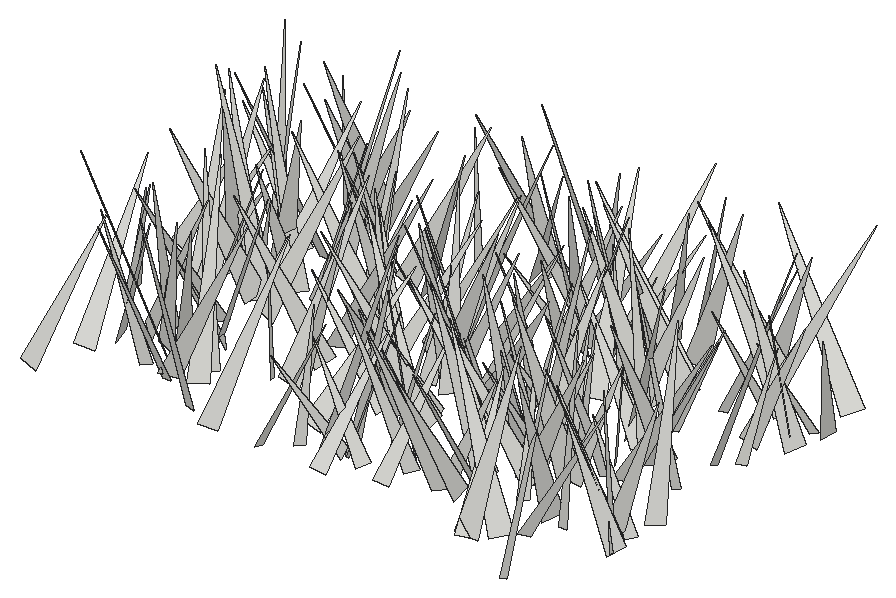
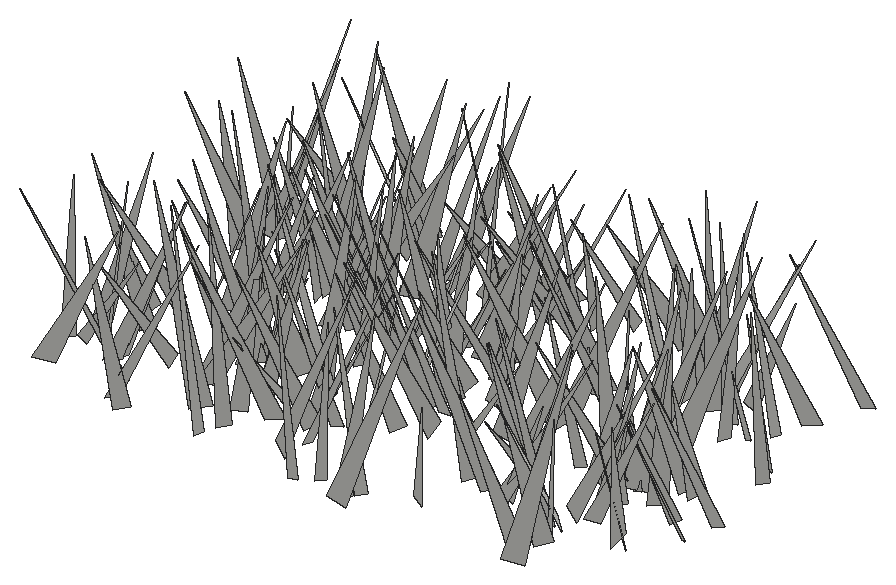
# SketchUp Ruby script. Lengths in inches.
U = 1.inch
M = Sketchup.active_model
def pt(a) = Geom::Point3d.new(a.map { |v| v * U })
def face(e, loops, mat)
  f = e.add_face(loops[0].map { |a| pt(a) })
  loops[1..].each { |l| e.add_face(l.map { |a| pt(a) }).erase! }
  f.material = f.back_material = mat if mat
  f
end
# faces: each face lists its corners as indices into pts; further lists are holes
def faces(e, pts, list, mat = nil) = list.each { |f| face(e, (f[0].is_a?(Array) ? f : [f]).map { |l| l.map { |i| pts[i] } }, mat) }
# xy, xz, yz: faces in a plane at the given z, y or x. An outline is a flat list of corners, or four numbers for a rectangle; further outlines are holes
def ring(l) = l.size == 4 ? [[l[0], l[1]], [l[2], l[1]], [l[2], l[3]], [l[0], l[3]]] : l.each_slice(2).to_a
def flat(e, list, mat, &to3) = list.each { |f| face(e, (f[0].is_a?(Array) ? f : [f]).map { |l| ring(l).map { |u, v| to3.(u, v) } }, mat) }
def xy(e, z, list, mat = nil) = flat(e, list, mat) { |x, y| [x, y, z] }
def xz(e, y, list, mat = nil) = flat(e, list, mat) { |x, z| [x, y, z] }
def yz(e, x, list, mat = nil) = flat(e, list, mat) { |y, z| [x, y, z] }
def lines(e, pts, list) = list.each { |a, b| e.add_line(pt(pts[a]), pt(pts[b])) }
# prism: a flat outline (further loops are holes) pulled along v
def prism(e, loops, v, mat = nil)
  f = face(e, loops, mat); d = Geom::Vector3d.new(v.map { |x| x * U })
  f.pushpull(f.normal.samedirection?(d) ? d.length : -d.length)
end
def box(e, o, s, mat = nil) = prism(e, [[o, [o[0] + s[0], o[1], o[2]], [o[0] + s[0], o[1] + s[1], o[2]], [o[0], o[1] + s[1], o[2]]]], [0, 0, s[2]], mat)
def at(x, y, z, deg = 0) = Geom::Transformation.translation(pt([x, y, z])) * Geom::Transformation.rotation(ORIGIN, Z_AXIS, deg.degrees)
def axes(o, x, y, z) = Geom::Transformation.new([*x, 0, *y, 0, *z, 0, *pt(o).to_a, 1])
def part(name) = M.definitions.add(name)
# library, detail: a bought-in or finely detailed component or shape, given as its bounding box
def library(name, o, s) = part(name).tap { |d| box(d.entities, o, s) }
def detail(e, o, s) = box(e.add_group.entities, o, s)
def put(e, d, t, mat = nil) = e.add_instance(d, t).tap { |i| i.material = mat if mat }
def group(e, t, mat = nil) = e.add_group.tap { |g| g.transformation = t; g.material = mat if mat }.entities
root = M.entities
c1 = part("fur_instance\#9")
p = [[0.8125,0,1.79],[0.67,-0.02,1.48],[0,-0.11,0],[0,0.11,0]]
faces(c1.entities,p,[[0,1,2,3]])
put(root,c1,axes([534.58,361.02,-21.66],[-6.04066,-0.63869,2.51357],[0.73038,5.69455,3.20222],[2.48847,-3.22176,5.16172]))
put(root,c1,axes([538.41,356.86,-21.66],[-1.59502,6.99566,2.35908],[7.02793,2.17795,-1.70682],[2.26111,-1.83463,6.96922]))
put(root,c1,axes([525,360.51,-21.66],[-5.02387,-1.18033,0.42976],[-0.88594,4.58548,2.23734],[0.8905,-2.09699,4.65046]))
put(root,c1,axes([538.34,359.93,-21.66],[-2.23247,-5.83337,0.18602],[-5.6892,2.13065,-1.46288],[-1.30221,0.692,6.07224]))
put(root,c1,axes([543.93,353.875,-21.66],[4.35175,7.0169,0.44581],[6.16578,-4.0605,3.72408],[-3.37917,1.6275,7.36925]))
put(root,c1,axes([500.89,356.83,-21.66],[0.65701,6.39206,0.99008],[6.12037,-0.29236,-2.17392],[2.09278,-1.15171,6.04683]))
put(root,c1,axes([533.23,360.72,-21.66],[1.95168,-6.84621,1.26966],[-6.52036,-2.2596,-2.16121],[-2.44285,0.56154,6.78298]))
put(root,c1,axes([513.05,358.93,-21.66],[-3.81075,-5.76969,1.72606],[-6.01138,3.52106,-1.50194],[-0.36316,2.25903,6.74947]))
put(root,c1,axes([540.23,358.26,-21.66],[-4.97351,5.86998,1.15657],[5.9442,4.67754,1.82131],[-0.6788,-2.04794,7.47498]))
put(root,c1,axes([538.38,356.68,-21.66],[-4.13598,4.27474,0.09369],[4.07434,3.97972,-1.71759],[1.29691,1.13001,5.6947]))
put(root,c1,axes([519.9,357.75,-21.66],[4.92859,0.75105,0.39032],[0.57555,-4.66461,1.7081],[-0.62062,1.63853,4.68375]))
put(root,c1,axes([541.375,362.4,-21.66],[6.17469,-3.94346,0.96595],[-3.5616,-6.10514,-2.15707],[-1.94909,-1.33681,7.00177]))
put(root,c1,axes([527.08,360,-21.66],[-3.88127,2.88585,0.74535],[2.95869,3.58243,1.53633],[-0.36036,-1.66913,4.58608]))
put(root,c1,axes([509.43,361.02,-21.66],[-2.97,-5.19915,0.68344],[-5.09037,2.66981,-1.8109],[-1.25951,1.46972,5.70725]))
put(root,c1,axes([547.59,361.41,-21.66],[-5.95975,2.47486,1.75961],[2.91321,5.75356,1.77469],[0.85695,-2.34763,6.20435]))
put(root,c1,axes([546.71,363.14,-21.66],[-5.73536,-5.62008,0.65862],[-5.46135,5.74328,1.44982],[1.48081,-0.58562,7.89796]))
put(root,c1,axes([525.1,357.56,-21.66],[-2.44099,4.81015,0.04297],[4.37742,2.2412,-2.21652],[1.99437,0.96814,4.91762]))
put(root,c1,axes([521.98,359.56,-21.66],[-4.57761,1.25738,1.06742],[0.91701,4.55759,-1.43608],[1.37093,1.14988,4.52473]))
put(root,c1,axes([528.41,363.76,-21.66],[-4.91582,-6.36103,2.07601],[-5.8042,5.33544,2.60426],[3.32923,-0.09063,7.60565]))
put(root,c1,axes([515.68,357.57,-21.66],[-5.17652,4.83446,1.05401],[3.91261,4.93311,-3.41105],[3.02894,1.88989,6.20751]))
put(root,c1,axes([527.79,361.93,-21.66],[5.79589,4.16761,1.50359],[4.42839,-5.37215,-2.17978],[0.13803,-2.64446,6.79779]))
put(root,c1,axes([508.77,363.5,-21.66],[7.2919,-1.58164,0.56037],[-1.39543,-7.10365,-1.89164],[-0.93186,-1.73896,7.21769]))
put(root,c1,axes([541.37,359.32,-21.66],[5.52796,-0.81869,0.7417],[-1.07099,-4.89962,2.57397],[-0.27083,2.66498,4.96017]))
put(root,c1,axes([530.12,361.35,-21.66],[-1.81659,5.58818,1.87966],[5.39696,0.78429,2.88421],[-2.37355,-2.49359,5.11948]))
put(root,c1,axes([509.28,361.95,-21.66],[-6.03257,-5.76703,0.56772],[-5.59645,5.58532,-2.7307],[-1.50355,2.34912,7.8863]))
put(root,c1,axes([509.28,361.45,-21.66],[5.54301,-4.89223,1.08245],[-4.92161,-5.01325,2.54471],[0.93987,2.60075,6.94141]))
put(root,c1,axes([529.46,358.88,-21.66],[-3.68567,4.23937,0.30212],[3.60627,3.33103,-2.74713],[2.24908,1.60613,4.89997]))
put(root,c1,axes([507.11,361.72,-21.66],[-0.49335,5.1966,1.87912],[5.02115,-0.36617,2.33091],[-2.30734,-1.90798,4.67065]))
put(root,c1,axes([524.16,359.375,-21.66],[7.79418,1.63756,2.08164],[0.8535,-7.67768,2.8441],[-2.50726,2.47704,7.43922]))
put(root,c1,axes([547.46,361.1875,-21.66],[-5.30333,-1.20318,1.41609],[-1.56427,5.2022,-1.4382],[1.00301,1.75149,5.24448]))
put(root,c1,axes([503.37,363.69,-21.66],[6.27835,0.76334,0.54412],[0.88551,-6.03847,-1.74618],[-0.30762,-1.80294,6.07875]))
put(root,c1,axes([506.75,364.37,-21.66],[-0.2881,-6.79413,1.19024],[-6.52945,0.65262,2.14482],[2.22333,1.03623,6.45314]))
put(root,c1,axes([532.37,362.93,-21.66],[1.52627,-4.48364,1.33128],[-4.39877,-0.90019,2.01128],[1.58937,1.81423,4.28804]))
put(root,c1,axes([545.87,363.15,-21.66],[3.29636,-5.4576,1.30622],[-5.51274,-2.86598,1.93739],[1.04942,2.08768,6.07437]))
put(root,c1,axes([525.49,360.79,-21.66],[-6.79191,0.51616,3.38033],[-0.49773,7.28774,-2.11287],[3.3831,2.10844,6.47551]))
put(root,c1,axes([534.21,364.12,-21.66],[4.0303,-5.81988,3.12764],[-5.66664,-4.92868,-1.86917],[-3.39741,1.31665,6.82792]))
put(root,c1,axes([525.58,360.23,-21.66],[4.27823,3.00126,0.70858],[2.21616,-3.83495,2.86263],[-2.14435,2.02448,4.3722]))
put(root,c1,axes([547.22,363.49,-21.66],[-1.85647,3.95367,0.8299],[3.82368,1.42492,1.76516],[-1.30372,-1.4508,3.99527]))
put(root,c1,axes([542.79,361.7,-21.66],[2.80201,6.02167,1.40008],[5.6342,-3.12002,2.14317],[-2.54489,-0.27744,6.28638]))
put(root,c1,axes([502.4,360.99,-21.66],[-2.48989,6.58556,0.19317],[6.42005,2.47161,-1.51018],[1.47984,0.3578,6.87667]))
put(root,c1,axes([536.97,365.12,-21.66],[3.33833,-6.51025,0.54896],[-6.14625,-2.92038,2.74304],[2.21549,1.70799,6.78259]))
put(root,c1,axes([537.54,365.03,-21.66],[-4.43221,4.72995,1.58971],[4.78005,3.41433,3.16821],[-1.43205,-3.24253,5.65503]))
put(root,c1,axes([504.45,365.29,-21.66],[5.46808,5.3055,1.78388],[5.41419,-4.38056,-3.56761],[1.42026,-3.72732,6.73205]))
put(root,c1,axes([505.75,366.23,-21.66],[6.82649,-0.20783,2.36031],[0.47416,-6.93274,-1.9818],[-2.32152,-2.02711,6.5358]))
put(root,c1,axes([524.76,367.15,-21.66],[3.41213,-4.67618,0.33772],[-4.46229,-3.36731,-1.54031],[-1.43828,-0.64649,5.58003]))
put(root,c1,axes([539.12,367.1,-21.66],[5.28612,-6.00356,2.19792],[-5.60526,-5.72373,-2.15328],[-3.07484,0.113,7.70384]))
put(root,c1,axes([536.71,367.59,-21.66],[-4.92711,-3.11526,0.5387],[-2.69685,4.66208,2.29422],[1.64986,-1.68274,5.3589]))
put(root,c1,axes([509.4375,367.28,-21.66],[-3.6044,-3.37024,0.34721],[-3.01204,3.4196,1.92476],[1.55135,-1.19103,4.54373]))
put(root,c1,axes([538.32,363.05,-21.66],[-4.43133,1.84787,0.51045],[1.62369,4.30117,-1.47494],[1.01922,1.18203,4.56901]))
put(root,c1,axes([521.04,362.04,-21.66],[-1.51427,6.54379,0.36236],[5.84338,1.51647,-2.96661],[2.96773,0.35306,6.02606]))
put(root,c1,axes([511.43,361.89,-21.66],[-6.67493,4.02137,0.12146],[3.83511,6.43107,-2.16198],[1.21576,1.79188,7.48679]))
put(root,c1,axes([527.21,367.38,-21.66],[-8.16776,0.06376,0.0825],[0.08376,7.86119,2.21763],[0.06209,-2.2183,7.8612]))
put(root,c1,axes([539.56,364.4,-21.66],[-6.70794,-1.60484,0.19836],[-1.59675,6.44001,-1.8942],[-0.25542,1.88735,6.63204]))
put(root,c1,axes([508.95,367.23,-21.66],[8.07507,1.50255,0.4439],[1.56674,-7.73574,-2.31627],[0.00564,-2.35841,7.88031]))
put(root,c1,axes([522.47,369.46,-21.66],[4.86562,-4.5964,0.06859],[-4.19123,-4.47675,-2.68294],[-1.88818,-1.90726,6.13213]))
put(root,c1,axes([507.2,369.33,-21.66],[2.70234,-6.75975,0.1599],[-6.39067,-2.60962,-2.31767],[-2.20886,-0.71979,6.90111]))
put(root,c1,axes([511.02,363.67,-21.66],[-7.30125,2.0292,0.54339],[1.84392,7.1322,-1.85816],[1.00641,1.65384,7.34664]))
put(root,c1,axes([533.92,368.34,-21.66],[4.85347,-3.26157,0.26621],[-3.0891,-4.72355,-1.55255],[-1.07988,-1.1468,5.6377]))
put(root,c1,axes([516.47,366.8,-21.66],[3.82304,5.79974,2.60132],[6.29108,-3.01834,-2.51622],[0.9089,-3.50316,6.47466]))
put(root,c1,axes([523.32,366.76,-21.66],[-5.14523,1.96025,0.06602],[1.88898,4.90265,1.64806],[-0.52792,-1.56261,5.25356]))
put(root,c1,axes([514.91,365.48,-21.66],[-3.90269,-1.36809,1.23152],[-1.73858,3.68797,-1.41263],[0.60468,1.77384,3.88679]))
put(root,c1,axes([536.375,366.77,-21.66],[2.73482,-5.11249,1.4467],[-5.08402,-2.04521,2.38319],[1.54377,2.32148,5.28557]))
put(root,c1,axes([516.375,369.32,-21.66],[-6.66712,2.68909,2.42043],[3.53397,5.92752,3.14894],[0.77508,-3.89533,6.46266]))
put(root,c1,axes([500.76,367.66,-21.66],[-1.89095,-4.65132,2.366],[-4.60338,2.67208,1.57395],[2.45798,1.42605,4.76793]))
put(root,c1,axes([539.4,366.96,-21.66],[-0.77235,4.89048,2.70767],[4.92537,1.88806,-2.00519],[2.64368,-2.08884,4.52687]))
put(root,c1,axes([526.59,368.86,-21.66],[-3.56897,-0.50146,0.42511],[-0.28446,3.29362,1.49696],[0.59267,-1.43888,3.27843]))
put(root,c1,axes([533.05,368.97,-21.66],[-6.0404,2.2493,3.21945],[3.13358,6.3206,1.46334],[2.36747,-2.62704,6.2773]))
put(root,c1,axes([499.96,369.28,-21.66],[5.73315,-1.08828,0.33068],[-0.98004,-5.58896,-1.40205],[-0.57725,-1.3198,5.66459]))
put(root,c1,axes([516.2,365.64,-21.66],[0.38295,8.08113,1.09098],[7.9956,-0.1576,-1.6392],[1.60161,-1.14545,7.92239]))
put(root,c1,axes([547.3125,365.94,-21.66],[-5.92088,3.75972,1.43779],[3.50525,6.07307,-1.44586],[1.97886,0.49178,6.86307]))
put(root,c1,axes([540.71,368.97,-21.66],[-1.01411,-6.0227,1.51425],[-5.97973,0.53295,-1.88497],[-1.67593,1.7428,5.80932]))
put(root,c1,axes([536.11,370.92,-21.66],[3.38656,-3.48151,1.0277],[-2.77448,-3.38882,-2.33752],[-2.3408,-1.02022,4.25743]))
put(root,c1,axes([525.11,367.82,-21.66],[-3.78872,6.01371,0.63065],[5.87535,3.48538,2.06137],[-1.42923,-1.61377,6.8022]))
put(root,c1,axes([530.73,369.39,-21.66],[-3.83855,4.56526,0.77541],[4.17711,2.97899,3.13921],[-1.99865,-2.54191,5.07163]))
put(root,c1,axes([538.84,367.01,-21.66],[-5.03448,1.97141,0.87824],[1.57247,4.87743,-1.93439],[1.47821,1.52579,5.04882]))
put(root,c1,axes([541.9,369.2,-21.66],[6.07863,-4.42165,0.21276],[-4.21796,-5.67554,2.55792],[1.3435,2.18706,7.06807]))
put(root,c1,axes([539.06,367.86,-21.66],[-5.01986,0.40192,1.5189],[-0.17545,4.90978,-1.87904],[1.56135,1.84392,4.67223]))
put(root,c1,axes([526.98,372.4,-21.66],[-6.21102,-4.85766,0.88936],[-4.64444,6.23147,1.60082],[1.67841,-0.73247,7.72082]))
put(root,c1,axes([539.78,371.12,-21.66],[4.17117,1.8451,1.43695],[2.27213,-3.89306,-1.59669],[-0.55375,-2.07548,4.27243]))
put(root,c1,axes([530.96,368.66,-21.66],[-6.11447,-3.98639,0.59028],[-3.68819,5.10346,-3.73879],[-1.62389,3.41906,6.26894]))
put(root,c1,axes([505.19,371.05,-21.66],[6.89965,2.05968,0.48381],[2.11498,-6.67017,-1.76557],[0.05673,-1.82978,6.98071]))
put(root,c1,axes([528.01,372.39,-21.66],[1.13503,-7.67663,0.6742],[-6.50823,-0.58999,4.2389],[4.12651,1.18099,6.50005]))
put(root,c1,axes([515.25,367.24,-21.66],[6.25178,5.32919,0.93445],[4.93149,-6.20008,2.36594],[-2.22574,1.23164,7.86685]))
put(root,c1,axes([542.48,373.15,-21.66],[3.73251,-5.71066,0.85994],[-5.41751,-3.81707,-1.83396],[-2.00044,-0.31799,6.57114]))
put(root,c1,axes([534.16,367.86,-21.66],[3.4696,4.95294,0.18512],[4.68916,-3.35343,1.83583],[-1.60551,0.90933,5.7619]))
put(root,c1,axes([507.08,373.47,-21.66],[-7.12654,1.94071,2.81889],[3.04033,6.57978,3.15641],[1.57127,-3.9294,6.67765]))
put(root,c1,axes([522.04,369.34,-21.66],[-6.81045,0.95525,0.6863],[0.79996,6.71798,-1.4123],[0.86231,1.31226,6.73054]))
put(root,c1,axes([523.93,373.36,-21.66],[5.76412,-4.56343,1.38579],[-4.26746,-5.90574,-1.69745],[-2.12934,-0.51736,7.15322]))
put(root,c1,axes([535.9,367.22,-21.66],[7.29611,1.84526,3.54482],[-0.04664,-7.33917,3.91643],[-3.99607,3.45479,6.4265]))
put(root,c1,axes([534.38,369.73,-21.66],[-2.83058,6.09964,1.95872],[5.76034,3.3604,-2.14023],[2.80369,-0.74599,6.37473]))
put(root,c1,axes([531.0625,373.53,-21.66],[5.81845,-0.62274,2.18855],[-0.03101,-6.03017,-1.6334],[-2.27522,-1.51035,5.61909]))
put(root,c1,axes([523.18,373.42,-21.66],[5.01421,-5.55154,0.43768],[-5.45899,-4.78379,1.86233],[1.10028,1.565,7.24525]))
put(root,c1,axes([545.39,370.61,-21.66],[-6.80362,-1.51626,0.05987],[-1.39466,6.13985,-2.9915],[-0.59797,2.93174,6.29597]))
put(root,c1,axes([520.3,370.92,-21.66],[1.42855,6.69806,0.59183],[6.31436,-1.12829,-2.47201],[2.31152,-1.05735,6.38701]))
put(root,c1,axes([515.41,371.52,-21.66],[7.23014,-2.66142,0.8801],[-2.79977,-6.73645,2.62947],[0.1379,2.76941,7.24182]))
put(root,c1,axes([538.4,374.62,-21.66],[7.85727,-0.11013,0.63762],[0.0287,-7.70188,-1.68396],[-0.64642,-1.6806,7.67549]))
put(root,c1,axes([527.13,372.38,-21.66],[4.92095,5.18553,0.33695],[5.09859,-4.72846,-1.69263],[1.00379,-1.4039,6.94554]))
put(root,c1,axes([525.42,371.26,-21.66],[-6.65914,2.85732,1.17721],[2.6023,6.69305,-1.52492],[1.66678,0.96593,7.084]))
put(root,c1,axes([541.93,371.97,-21.66],[5.39304,-0.33096,0.39775],[-0.43435,-5.15892,1.59671],[-0.28121,1.6213,5.16187]))
put(root,c1,axes([509.06,371.89,-21.66],[1.74287,7.71217,1.36191],[7.45298,-1.20484,-2.71503],[2.4053,-1.85492,7.42588]))
put(root,c1,axes([503.64,375.98,-21.66],[7.57168,-2.77915,1.4038],[-2.39268,-7.55557,-2.05259],[-1.99233,-1.48808,7.80006]))
put(root,c1,axes([539.83,373.61,-21.66],[-4.53112,4.00144,0.54603],[3.94801,4.21612,1.86503],[-0.85024,-1.74745,5.75015]))
put(root,c1,axes([526.09,373.76,-21.66],[-5.87124,-3.56524,0.53214],[-3.58838,5.68376,-1.51131],[-0.34307,1.5651,6.70063]))
put(root,c1,axes([520.78,372.16,-21.66],[-1.18961,5.30841,0.21099],[4.92708,1.02155,2.07828],[-1.98686,-0.64508,5.02744]))
put(root,c1,axes([510.92,375.14,-21.66],[-0.06945,-5.66946,1.63507],[-5.27402,0.7929,2.5253],[2.64594,1.43164,5.07647]))
put(root,c1,axes([531.5,377.09,-21.66],[5.49992,-4.64771,0.52674],[-4.40214,-5.41809,-1.84207],[-1.58109,-1.08206,6.96111]))
put(root,c1,axes([505.89,375.27,-21.66],[-0.58442,-4.16845,1.10453],[-3.96593,0.95723,1.51414],[1.69333,0.80327,3.92746]))
put(root,c1,axes([517.53,375.21,-21.66],[-1.28539,6.13898,3.44989],[6.89976,0.39684,1.86462],[-1.40785,-3.66012,5.98853]))
put(root,c1,axes([515.48,375.9,-21.66],[-6.93796,2.79801,1.11968],[3.01121,6.55067,2.28891],[0.12298,-2.54512,7.12215]))
put(root,c1,axes([506.13,375.28,-21.66],[-4.3642,6.37446,3.0679],[7.06974,4.05938,1.62241],[0.25406,-3.46117,7.553]))
put(root,c1,axes([523.39,371.46,-21.66],[-6.0414,2.82747,0.77084],[2.14541,5.47009,-3.25002],[1.99649,2.67784,5.82499]))
put(root,c1,axes([540.51,373.5,-21.66],[-7.44461,1.33123,0.56849],[1.18187,7.30967,-1.63995],[0.83578,1.52121,7.38274]))
put(root,c1,axes([506.66,377.63,-21.66],[4.42124,-3.27,0.9733],[-2.9097,-4.44582,-1.71927],[-1.78153,-0.85401,5.22344]))
put(root,c1,axes([523.77,374.9375,-21.66],[4.38543,-2.43855,0.87514],[-2.59033,-4.09309,1.5752],[0.05089,1.80126,4.76417]))
put(root,c1,axes([507.56,373.45,-21.66],[-0.98442,7.82804,0.7856],[7.24103,0.59195,3.17514],[-3.07617,-1.11168,7.22258]))
put(root,c1,axes([520.4375,374.95,-21.66],[4.59981,5.90875,0.46757],[5.722,-4.27232,-2.30133],[1.54616,-1.76752,7.12569]))
put(root,c1,axes([503.27,372.98,-21.66],[-5.30404,4.85737,1.41696],[4.30663,5.41145,-2.42976],[2.65607,0.92563,6.76928]))
put(root,c1,axes([505.93,377.67,-21.66],[3.30529,-7.09092,0.75642],[-7.06387,-3.14139,1.41833],[0.97724,1.27626,7.69379]))
put(root,c1,axes([502.29,373.39,-21.66],[-5.42402,3.35952,0.54018],[3.08821,5.28712,-1.87283],[1.42868,1.32596,6.09909]))
put(root,c1,axes([522.53,375.12,-21.66],[2.40606,6.39383,1.08481],[6.38564,-2.13376,-1.58675],[1.13207,-1.55339,6.64473]))
put(root,c1,axes([498.61,375.78,-21.66],[0.87918,5.14411,1.43079],[4.85097,-0.16366,-2.39235],[2.23095,-1.67133,4.63805]))
put(root,c1,axes([536.82,376.69,-21.66],[-2.52237,2.99386,0.77548],[2.99232,2.10973,1.58806],[-0.78138,-1.58517,3.57821]))
put(root,c1,axes([540.13,376.57,-21.66],[4.26333,-3.02404,0.31767],[-2.97687,-4.03955,1.49732],[0.61963,1.39963,5.00788]))
put(root,c1,axes([519.09,377.5625,-21.66],[-2.36065,-3.34559,0.0438],[-3.13879,2.19578,-1.44709],[-1.15883,0.86782,3.83035]))
put(root,c1,axes([501.26,377.03,-21.66],[2.74116,-2.85153,0.16279],[-2.64199,-2.44575,1.64616],[1.08517,1.2485,3.59657]))
put(root,c1,axes([537.125,378.0625,-21.66],[-7.26006,2.55391,1.83228],[2.95803,7.11093,1.80912],[1.0629,-2.34529,7.48051]))
put(root,c1,axes([529.85,378.1,-21.66],[8.09633,1.85359,0.38508],[1.89305,-7.94545,-1.5559],[-0.02113,-1.6027,8.15877]))
put(root,c1,axes([536.59,377.41,-21.66],[1.17731,-6.81979,2.88625],[-6.91612,0.0321,2.89694],[2.64712,3.11697,6.28517]))
put(root,c1,axes([546.7,375.9,-21.66],[3.7026,-0.58317,1.91769],[-1.4169,-3.61072,1.63767],[-1.41775,2.08554,3.37155]))
put(root,c1,axes([508.91,375.88,-21.66],[-0.71343,7.62578,1.29035],[7.14993,0.15622,3.02994],[-2.94889,-1.46615,7.03427]))
put(root,c1,axes([545.24,378.44,-21.66],[1.83372,-5.8574,1.52699],[-5.60076,-1.03656,2.74963],[2.29617,2.14936,5.48737]))
put(root,c1,axes([525.13,380.38,-21.66],[-2.98193,-4.15353,0.46379],[-3.81224,2.9367,1.78925],[1.71281,-0.69483,4.78981]))
put(root,c1,axes([523.67,378.67,-21.66],[3.57334,-4.4658,0.19156],[-4.12422,-3.19939,2.34597],[1.72363,1.60293,5.21618]))
put(root,c1,axes([507.09,375.42,-21.66],[-0.93463,7.10607,0.24964],[6.82555,0.96718,-1.97702],[1.99262,0.02006,6.88921]))
put(root,c1,axes([536.3125,376.34,-21.66],[-5.7713,0.32455,0.04644],[0.28097,5.31808,-2.2482],[0.16895,2.24233,5.3253]))
put(root,c1,axes([545.32,374.75,-21.66],[6.83312,3.40706,1.30672],[2.45514,-6.34476,3.70451],[-2.69961,2.8536,6.67654]))
put(root,c1,axes([528.7,380.93,-21.66],[-4.92347,-1.39259,0.14711],[-1.23579,4.5738,1.93769],[0.65861,-1.82825,4.73553]))
put(root,c1,axes([507.3,377.36,-21.66],[-6.47288,0.26814,0.01301],[0.25719,6.28405,-1.55397],[0.07694,1.55212,6.2893]))
put(root,c1,axes([548.21,379.76,-21.66],[-6.07802,2.92755,1.98205],[3.37511,5.97833,1.51972],[1.05246,-2.26504,6.57292]))
put(root,c1,axes([513.8,377.38,-21.66],[4.21835,1.12148,1.8478],[0.48542,-4.44001,1.58659],[-2.10629,1.22277,4.06632]))
put(root,c1,axes([499.32,378.64,-21.66],[3.29682,4.04593,0.27696],[3.82738,-2.98619,-1.93627],[1.34069,-1.42422,4.84659]))
put(root,c1,axes([507.35,380.53,-21.66],[-3.5976,-6.50533,0.64098],[-6.34012,3.29439,-2.15004],[-1.59153,1.58132,7.11613]))
put(root,c1,axes([534.4,379.27,-21.66],[0.81184,5.62301,2.88886],[5.96448,-1.64652,1.52868],[-2.09495,-2.50871,5.47179]))
put(root,c1,axes([515.63,381.12,-21.66],[7.87771,-0.03675,0.30438],[0.03502,-7.66773,-1.83222],[-0.30459,-1.83219,7.66177]))
put(root,c1,axes([538.15,380.98,-21.66],[-7.32197,2.2534,1.35544],[2.57225,6.97064,2.30649],[0.54639,-2.61889,7.30542]))
put(root,c1,axes([544.14,382.23,-21.66],[-5.03232,-2.4099,0.87584],[-1.92345,4.82363,2.22078],[1.6956,-1.68045,5.11859]))
put(root,c1,axes([546.28,381.51,-21.66],[-3.5454,-4.09399,1.47684],[-3.82101,3.83994,1.47185],[2.08366,0.07566,5.21193]))
put(root,c1,axes([521.68,377.29,-21.66],[7.63616,1.08232,1.22596],[0.61242,-7.3209,2.64853],[-1.51635,2.49367,7.24345]))
put(root,c1,axes([505.67,380.43,-21.66],[-4.20776,3.77593,1.0344],[3.85861,3.7428,2.0336],[-0.66241,-2.18328,5.27517]))
put(root,c1,axes([512.74,378.15,-21.66],[-3.04551,1.64304,1.0176],[0.80196,2.80235,-2.12461],[1.7584,1.56764,2.73144]))
put(root,c1,axes([513.96,376.95,-21.66],[-7.01528,2.7432,0.95764],[2.14491,6.5776,-3.12905],[1.96,2.6204,6.85188]))
put(root,c1,axes([533.31,376.77,-21.66],[-6.01479,5.28528,0.0687],[5.03484,5.76049,-2.36301],[1.60915,1.73181,7.65037]))
put(root,c1,axes([533.56,383.39,-21.66],[5.51839,-2.97407,0.09463],[-2.75984,-5.19025,-2.17974],[-1.11235,-1.87694,5.87762]))
put(root,c1,axes([533.8125,380.1,-21.66],[0.77097,6.55392,2.92574],[6.60675,-1.79779,2.28627],[-2.8044,-2.43357,6.19042]))
put(root,c1,axes([548.8,382.6,-21.66],[5.13341,-1.95182,0.40555],[-1.78394,-4.9977,-1.47188],[-0.88973,-1.24068,5.29103]))
put(root,c1,axes([529.16,381.125,-21.66],[-3.64938,-5.29226,1.74557],[-5.55344,3.28039,-1.66476],[-0.463,2.36729,6.20923]))
put(root,c1,axes([527.09,380.93,-21.66],[1.94999,6.06367,1.85826],[6.06829,-1.21894,-2.39034],[1.84311,-2.40204,5.90397]))
put(root,c1,axes([512.32,381.87,-21.66],[-4.6508,-5.63712,0.37429],[-5.36466,4.25457,-2.58191],[-1.77136,1.91537,6.83673]))
put(root,c1,axes([527.18,383.97,-21.66],[-7.29024,-1.74958,0.87658],[-1.40156,7.02793,2.37084],[1.36568,-2.12702,7.11251]))
put(root,c1,axes([547.84,382.28,-21.66],[-0.53868,-3.7535,0.51973],[-3.36849,0.23389,-1.80211],[-1.73555,0.71104,3.33637]))
put(root,c1,axes([511.94,381.61,-21.66],[-1.05055,-3.99645,1.56356],[-4.12582,0.49771,-1.49997],[-1.18067,1.81677,3.85037]))
put(root,c1,axes([537.49,381.85,-21.66],[-6.42815,4.45601,0.04956],[4.21627,6.0534,2.59983],[-1.44275,-2.16333,7.37686]))
put(root,c1,axes([513.7,381.25,-21.66],[0.25719,7.17904,2.90731],[6.91163,1.10018,-3.3281],[3.49578,-2.70337,6.36621]))
put(root,c1,axes([528.39,381.92,-21.66],[4.87522,-3.55324,0.35007],[-3.38958,-4.41978,2.34354],[1.12198,2.08707,5.55888]))
put(root,c1,axes([544.53,383.12,-21.66],[-6.88709,2.46248,0.81316],[2.58785,6.67518,1.70354],[0.16756,-1.88022,7.11293]))
put(root,c1,axes([531.35,380.62,-21.66],[3.64416,1.65962,0.06909],[1.4569,-3.27351,1.789],[-0.79783,1.60274,3.58241]))
put(root,c1,axes([507.73,382.6,-21.66],[2.9133,6.77269,2.26525],[7.08174,-2.424,-1.8604],[0.9217,-2.7826,7.13411]))
put(root,c1,axes([507.59,385.87,-21.66],[5.40513,-4.44008,1.03103],[-3.91993,-5.34397,-2.46351],[-2.32626,-1.31164,6.54682]))
put(root,c1,axes([531.17,382.52,-21.66],[2.97178,5.39968,0.42783],[5.06638,-2.59832,-2.39825],[1.91609,-1.5044,5.67771]))
put(root,c1,axes([535.83,384.61,-21.66],[4.04324,-6.81137,0.9787],[-6.74817,-3.70246,2.11055],[1.34718,1.89668,7.63467]))
put(root,c1,axes([541.24,380.8,-21.66],[5.35308,0.77922,1.1136],[0.09871,-4.73607,2.83947],[-1.35556,2.73224,4.60435]))
put(root,c1,axes([533.02,385.6875,-21.66],[7.23074,-0.77372,0.74856],[-0.57311,-7.06946,-1.77111],[-0.91134,-1.69312,7.05304]))
put(root,c1,axes([506.23,384.91,-21.66],[2.55754,-6.5759,0.86107],[-6.14173,-2.00015,2.96707],[2.50263,1.81158,6.40156]))
put(root,c1,axes([502.31,381.33,-21.66],[3.51213,5.3509,1.08193],[4.75447,-3.63032,2.52063],[-2.68285,0.57134,5.88334]))
put(root,c1,axes([502.63,381.43,-21.66],[-7.06937,0.92542,0.80535],[0.55425,6.6114,-2.73188],[1.09444,2.62944,6.58553]))
put(root,c1,axes([506.96,383.36,-21.66],[2.66286,4.62658,1.9724],[4.32664,-3.24515,1.77077],[-2.56433,-0.67099,5.03592]))
put(root,c1,axes([530.92,382.8,-21.66],[-0.22471,7.89617,1.63504],[7.5306,0.79034,-2.78188],[2.88322,-1.44886,7.39332]))
put(root,c1,axes([506.36,388.0625,-21.66],[4.04445,-6.42376,0.8146],[-6.13253,-4.10829,-1.94934],[-2.07854,-0.37835,7.33638]))
put(root,c1,axes([507.27,381.95,-21.66],[4.44404,5.53922,0.27989],[5.13876,-4.2472,2.46279],[-2.08674,1.3376,6.66087]))
put(root,c1,axes([520.01,387.25,-21.66],[6.41369,-0.07562,0.05633],[-0.05586,-6.13403,-1.87481],[-0.07597,-1.87412,6.13403]))
put(root,c1,axes([523.32,387.39,-21.66],[5.23051,-1.10724,0.78196],[-0.81536,-5.06,-1.7109],[-1.08287,-1.53819,5.06527]))
put(root,c1,axes([528.1,385.8,-21.66],[-4.4516,-6.59475,1.62319],[-6.65602,3.85048,-2.61027],[-1.35017,2.76139,7.51625]))
put(root,c1,axes([507.82,385.99,-21.66],[4.10331,-3.61689,0.17449],[-3.47529,-3.85943,1.7253],[1.0172,1.40442,5.19061]))
put(root,c1,axes([533.65,387.55,-21.66],[7.53646,1.85279,1.2332],[2.16443,-7.11553,-2.53698],[-0.51849,-2.77277,7.33449]))
put(root,c1,axes([541.34,387.125,-21.66],[-6.98354,0.71492,0.27676],[0.75932,6.7998,1.59491],[0.10557,-1.6153,6.83646]))
put(root,c1,axes([520.72,389.03,-21.66],[0.06912,-7.57158,0.2529],[-7.42195,-0.11839,-1.51598],[-1.51902,0.23392,7.41859]))
put(root,c1,axes([520.83,388.11,-21.66],[5.55902,-2.83125,1.90418],[-2.404,-5.83322,-1.65498],[-2.42129,-0.70867,6.01496]))
put(root,c1,axes([542.3,384.78,-21.66],[3.82071,6.83533,0.31448],[6.59967,-3.58608,-2.23672],[1.80694,-1.35528,7.50444]))
put(root,c1,axes([548.06,386.11,-21.66],[-5.28258,5.45364,0.12335],[5.18528,4.96674,2.47132],[-1.69419,-1.80343,7.17917]))
put(root,c1,axes([516.51,385.55,-21.66],[1.26657,4.59176,1.22685],[4.36989,-1.62436,1.56816],[-1.86909,-0.68616,4.4977]))
put(root,c1,axes([539.9,388,-21.66],[2.36521,-5.47601,0.71506],[-5.30162,-2.03369,1.96193],[1.54624,1.40343,5.6331]))
put(root,c1,axes([524.92,388.42,-21.66],[-1.49518,-5.85947,1.8909],[-5.5495,2.12534,2.19783],[2.66683,1.13753,5.63369]))
